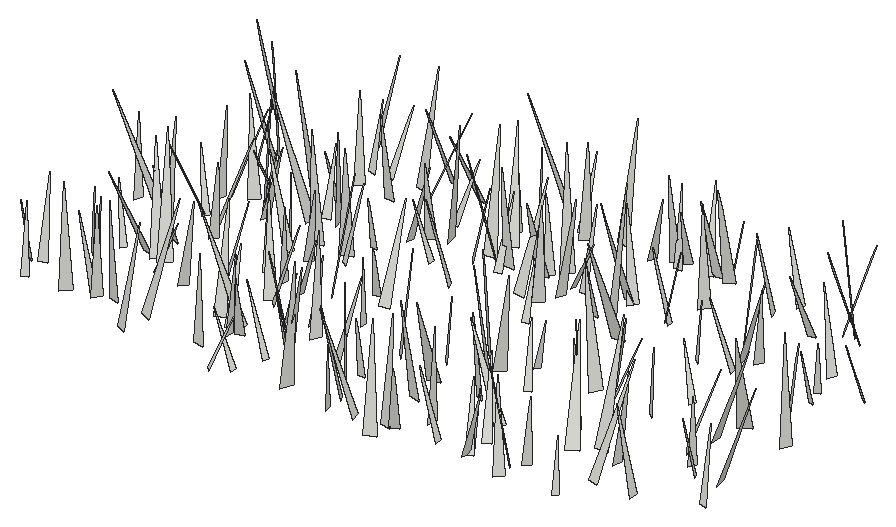
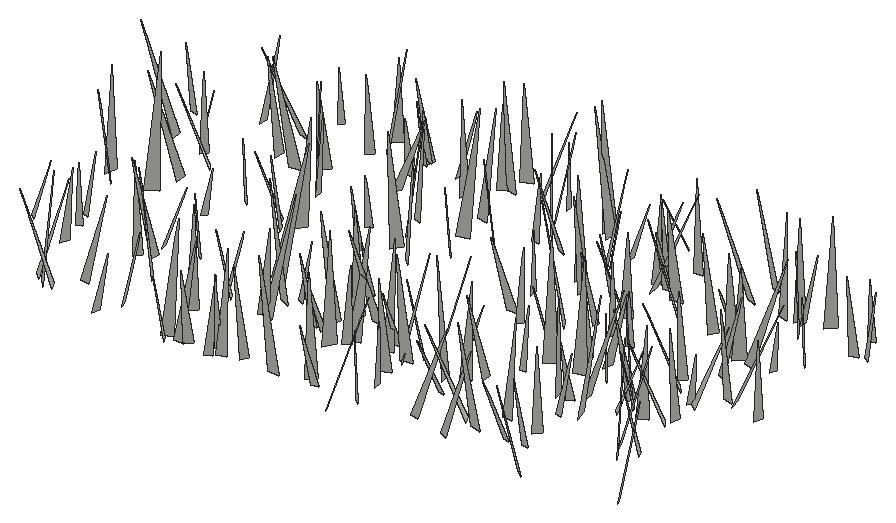
# SketchUp Ruby script. Lengths in inches.
U = 1.inch
M = Sketchup.active_model
def pt(a) = Geom::Point3d.new(a.map { |v| v * U })
def face(e, loops, mat)
  f = e.add_face(loops[0].map { |a| pt(a) })
  loops[1..].each { |l| e.add_face(l.map { |a| pt(a) }).erase! }
  f.material = f.back_material = mat if mat
  f
end
# faces: each face lists its corners as indices into pts; further lists are holes
def faces(e, pts, list, mat = nil) = list.each { |f| face(e, (f[0].is_a?(Array) ? f : [f]).map { |l| l.map { |i| pts[i] } }, mat) }
# xy, xz, yz: faces in a plane at the given z, y or x. An outline is a flat list of corners, or four numbers for a rectangle; further outlines are holes
def ring(l) = l.size == 4 ? [[l[0], l[1]], [l[2], l[1]], [l[2], l[3]], [l[0], l[3]]] : l.each_slice(2).to_a
def flat(e, list, mat, &to3) = list.each { |f| face(e, (f[0].is_a?(Array) ? f : [f]).map { |l| ring(l).map { |u, v| to3.(u, v) } }, mat) }
def xy(e, z, list, mat = nil) = flat(e, list, mat) { |x, y| [x, y, z] }
def xz(e, y, list, mat = nil) = flat(e, list, mat) { |x, z| [x, y, z] }
def yz(e, x, list, mat = nil) = flat(e, list, mat) { |y, z| [x, y, z] }
def lines(e, pts, list) = list.each { |a, b| e.add_line(pt(pts[a]), pt(pts[b])) }
# prism: a flat outline (further loops are holes) pulled along v
def prism(e, loops, v, mat = nil)
  f = face(e, loops, mat); d = Geom::Vector3d.new(v.map { |x| x * U })
  f.pushpull(f.normal.samedirection?(d) ? d.length : -d.length)
end
def box(e, o, s, mat = nil) = prism(e, [[o, [o[0] + s[0], o[1], o[2]], [o[0] + s[0], o[1] + s[1], o[2]], [o[0], o[1] + s[1], o[2]]]], [0, 0, s[2]], mat)
def at(x, y, z, deg = 0) = Geom::Transformation.translation(pt([x, y, z])) * Geom::Transformation.rotation(ORIGIN, Z_AXIS, deg.degrees)
def axes(o, x, y, z) = Geom::Transformation.new([*x, 0, *y, 0, *z, 0, *pt(o).to_a, 1])
def part(name) = M.definitions.add(name)
# library, detail: a bought-in or finely detailed component or shape, given as its bounding box
def library(name, o, s) = part(name).tap { |d| box(d.entities, o, s) }
def detail(e, o, s) = box(e.add_group.entities, o, s)
def put(e, d, t, mat = nil) = e.add_instance(d, t).tap { |i| i.material = mat if mat }
def group(e, t, mat = nil) = e.add_group.tap { |g| g.transformation = t; g.material = mat if mat }.entities
root = M.entities
c1 = part("fur_instance\#9")
p = [[0.8125,0,1.79],[0.67,-0.02,1.48],[0,-0.11,0],[0,0.11,0]]
faces(c1.entities,p,[[0,1,2,3]])
put(root,c1,axes([509.51,356.84,-21.66],[-2.53684,6.34204,1.9532],[6.60869,2.60398,0.12835],[0.60133,-1.86275,6.82939]))
put(root,c1,axes([486.03,357.42,-21.66],[2.19151,2.85606,0.09461],[2.85445,-2.18225,-0.24214],[0.13471,-0.22234,3.59182]))
put(root,c1,axes([510.63,359.85,-21.66],[2.81621,-4.35059,0.38195],[-4.36621,-2.81499,0.12899],[-0.09891,0.39082,5.18093]))
put(root,c1,axes([502.12,358.6,-21.66],[3.8396,0.83392,1.68617],[0.96833,-4.16197,-0.14664],[-1.61273,-0.51356,3.92638]))
put(root,c1,axes([505.58,359.22,-21.66],[-6.60705,-1.5953,0.55499],[-1.61141,6.62494,-0.14037],[0.50631,0.26714,6.79547]))
put(root,c1,axes([488.34,358.98,-21.66],[-3.79909,0.62191,0.11225],[0.62576,3.79759,0.13861],[0.08831,-0.15497,3.84716]))
put(root,c1,axes([526.51,358.57,-21.66],[-4.60516,3.74944,1.60687],[3.84875,4.79672,-0.16237],[1.35183,-0.88372,5.93628]))
put(root,c1,axes([472.625,358.48,-21.66],[2.70818,5.99392,1.73773],[6.22026,-2.74585,-0.22279],[-0.5051,-1.67756,6.57356]))
put(root,c1,axes([534.09,359.27,-21.66],[2.31719,-2.3997,1.71249],[-2.74416,-2.55172,0.13746],[-1.07739,1.33819,3.33302]))
put(root,c1,axes([520.69,360.01,-21.66],[4.88822,-0.89007,0.63341],[-0.87396,-4.92864,-0.18113],[-0.65546,-0.06625,4.96529]))
put(root,c1,axes([495.4,359.7,-21.66],[7.52534,-2.11015,2.94691],[-2.32099,-8.02168,0.183],[-2.78389,0.98374,7.81345]))
put(root,c1,axes([509.59,359.5625,-21.66],[-1.17344,-6.36654,3.3674],[-7.15717,1.41187,0.17527],[0.80444,3.27459,6.4714]))
put(root,c1,axes([516.35,360.58,-21.66],[-4.66446,-0.17714,0.77084],[-0.14932,4.72517,0.1823],[0.77671,-0.15541,4.66426]))
put(root,c1,axes([494.57,360.53,-21.66],[7.78387,0.2727,2.09642],[0.3333,-8.05673,-0.18953],[-2.08764,-0.26953,7.78634]))
put(root,c1,axes([525.74,361.49,-21.66],[4.20893,3.73459,3.7879],[4.59902,-4.98198,-0.19834],[-2.67289,-2.69131,5.62342]))
put(root,c1,axes([501.75,361.46,-21.66],[-4.7875,-3.33897,1.34753],[-3.4677,4.87923,-0.23006],[0.96934,0.96392,5.83232]))
put(root,c1,axes([481.63,361.12,-21.66],[0.33576,5.45677,2.6197],[6.05197,-0.25349,-0.24764],[0.11336,-2.62894,5.46148]))
put(root,c1,axes([520.93,360.85,-21.66],[1.65832,3.59632,1.35209],[3.82471,-1.68517,-0.20869],[-0.36513,-1.31848,3.95475]))
put(root,c1,axes([462.46,361.47,-21.66],[-4.98307,4.13485,3.06586],[4.6284,5.46651,0.15019],[2.25263,-2.08511,6.47344]))
put(root,c1,axes([521.05,360.26,-21.66],[-1.86481,4.13252,0.34952],[4.14724,1.85655,0.17621],[-0.01744,-0.39104,4.53037]))
put(root,c1,axes([456.92,361.08,-21.66],[-1.17354,4.22506,1.16991],[4.38332,1.15287,0.2334],[0.0799,-1.19029,4.3788]))
put(root,c1,axes([466.07,362.47,-21.66],[4.61817,-3.87726,2.02523],[-4.05143,-4.90172,-0.14567],[-1.64942,1.18414,6.02822]))
put(root,c1,axes([527.37,362.58,-21.66],[-2.45808,3.26284,2.53045],[3.74921,2.99751,-0.22312],[1.72995,-1.86016,4.07903]))
put(root,c1,axes([468.05,363.0625,-21.66],[-1.72933,-6.01967,2.37326],[-6.41752,1.90965,0.16749],[0.82719,2.23073,6.26091]))
put(root,c1,axes([465.38,362.79,-21.66],[-4.97388,0.03891,0.99351],[0.0174,5.07103,-0.11152],[0.99411,0.10595,4.97278]))
put(root,c1,axes([513.2,363.39,-21.66],[5.69837,-0.41307,2.53776],[-0.52377,-6.22748,0.16244],[-2.51724,0.36068,5.71101]))
put(root,c1,axes([489.6875,363.09,-21.66],[-4.67921,0.76999,0.1435],[0.76372,4.67821,-0.1991],[0.17382,0.17327,4.73796]))
put(root,c1,axes([454.9,364.58,-21.66],[-2.14945,-3.42966,1.0737],[-3.50191,2.27993,0.27214],[0.80747,0.75821,4.03839]))
put(root,c1,axes([541.13,364.33,-21.66],[-5.71627,0.02456,1.51927],[0.09668,5.9079,0.26822],[1.51639,-0.28405,5.71003]))
put(root,c1,axes([483.88,365.71,-21.66],[1.95757,-4.55386,0.31612],[-4.56359,-1.94437,0.25034],[0.10577,0.38911,4.95045]))
put(root,c1,axes([473.11,362.37,-21.66],[2.96798,6.81466,1.03357],[6.887,-2.97737,-0.1458],[-0.27767,-1.00619,7.4315]))
put(root,c1,axes([499.75,364.73,-21.66],[4.37424,4.04681,2.79179],[4.54542,-4.75288,-0.23239],[-1.87347,-2.08284,5.95454]))
put(root,c1,axes([482.98,364.96,-21.66],[5.23095,-0.44242,1.6949],[-0.413,-5.49862,-0.16069],[-1.70231,-0.02548,5.24716]))
put(root,c1,axes([464.22,365.03,-21.66],[4.38059,2.58911,2.20412],[2.75267,-4.81057,0.18002],[-1.99611,-0.9519,5.08534]))
put(root,c1,axes([508.18,366.46,-21.66],[-1.31696,-6.51866,1.83434],[-6.75362,1.40125,0.13086],[0.49623,1.77078,6.64907]))
put(root,c1,axes([520.74,363.67,-21.66],[-2.1836,4.82414,0.14178],[4.82373,2.17653,0.23433],[-0.15514,-0.2257,5.29014]))
put(root,c1,axes([490.73,366.17,-21.66],[3.77255,3.78798,3.73229],[4.48771,-4.72284,0.25719],[-2.85294,-2.4201,5.33992]))
put(root,c1,axes([456.43,364.95,-21.66],[-1.35199,5.16754,1.66066],[5.39955,1.4549,-0.13134],[0.55327,-1.57128,5.33986]))
put(root,c1,axes([490.39,365.94,-21.66],[-3.18222,-1.83698,0.96818],[-1.93012,3.2701,-0.13938],[0.76583,0.60852,3.67173]))
put(root,c1,axes([500.37,366.75,-21.66],[0.0054,-4.02258,1.09842],[-4.16704,0.03516,0.14925],[0.15324,1.09787,4.01982]))
put(root,c1,axes([483.22,367.07,-21.66],[-7.85705,-0.88135,0.16267],[-0.88597,7.85465,-0.23661],[0.1352,0.25331,7.90278]))
put(root,c1,axes([535.55,364.12,-21.66],[2.14003,7.20036,0.0672],[7.19519,-2.14104,0.27303],[-0.28086,0.01341,7.50668]))
put(root,c1,axes([482.07,366.15,-21.66],[-0.89857,4.82904,0.37817],[4.8418,0.88433,0.21213],[-0.14006,-0.41036,4.90735]))
put(root,c1,axes([496.72,366.71,-21.66],[2.68485,5.08236,0.90598],[5.15716,-2.6868,-0.21076],[-0.23424,-0.9002,5.74408]))
put(root,c1,axes([519.68,367.41,-21.66],[-6.207,1.9177,0.03314],[1.91765,6.20287,0.22937],[-0.03607,-0.22893,6.49244]))
put(root,c1,axes([507.38,370.92,-21.66],[2.10072,-7.09935,0.00934],[-7.09522,-2.09917,0.25546],[0.24231,0.08144,7.39923]))
put(root,c1,axes([548.48,367.56,-21.66],[0.70725,4.81258,1.31899],[4.97344,-0.78845,0.21001],[-0.40688,-1.27212,4.85974]))
put(root,c1,axes([479.67,367.54,-21.66],[-1.61925,6.67608,1.38838],[6.8184,1.60284,0.24489],[0.08425,-1.4073,6.86528]))
put(root,c1,axes([535.05,369.13,-21.66],[5.91491,-0.67607,1.90084],[-0.77835,-6.19702,0.21795],[-1.8613,0.44302,5.94943]))
put(root,c1,axes([459.38,370.02,-21.66],[3.09242,2.58599,1.68004],[2.84079,-3.31463,-0.12697],[-1.19992,-1.18273,4.02918]))
put(root,c1,axes([471.875,370.59,-21.66],[4.94298,-3.20176,1.42299],[-3.34359,-5.04595,0.26096],[-1.0472,0.99819,5.88356]))
put(root,c1,axes([529.19,368.38,-21.66],[-4.20767,6.2047,0.57896],[6.20765,4.23458,-0.26697],[0.54635,-0.32858,7.49209]))
put(root,c1,axes([491,370.375,-21.66],[-5.47966,3.19166,2.7493],[3.39794,6.01513,-0.2105],[2.48986,-1.18473,6.33791]))
put(root,c1,axes([513.71,371.15,-21.66],[-1.84582,-5.09705,1.94608],[-5.40108,1.99766,0.10933],[0.77171,1.78987,5.41987]))
put(root,c1,axes([486.34,370.81,-21.66],[3.55375,0.65284,0.74182],[0.70307,-3.6162,-0.18565],[-0.69441,-0.32026,3.60844]))
put(root,c1,axes([477.64,369.89,-21.66],[4.5925,4.65986,1.11021],[4.70947,-4.6734,0.13435],[-0.87619,-0.69491,6.5412]))
put(root,c1,axes([464.23,373.92,-21.66],[-1.51656,-6.50321,0.08888],[-6.50028,1.51258,-0.24097],[-0.21452,0.14123,6.67335]))
put(root,c1,axes([467.46,371.33,-21.66],[3.69637,0.13401,0.11411],[0.12786,-3.69317,0.19555],[-0.12096,0.19138,3.69362]))
put(root,c1,axes([489.01,372.57,-21.66],[4.9839,-2.53795,0.76874],[-2.53211,-5.04073,-0.2255],[-0.78777,0.14572,5.58834]))
put(root,c1,axes([543.72,372.26,-21.66],[-3.07283,-1.79032,0.75021],[-1.87261,3.10397,-0.26279],[0.51124,0.60869,3.54662]))
put(root,c1,axes([531.77,370.43,-21.66],[-0.24232,8.0833,1.63068],[8.24361,0.27788,-0.15248],[0.20433,-1.625,8.08549]))
put(root,c1,axes([527.19,372.4,-21.66],[-5.46878,-3.64969,2.6695],[-4.02035,5.84198,-0.2491],[2.0696,1.70441,6.57007]))
put(root,c1,axes([546.8,372.83,-21.66],[7.02887,1.41814,0.69885],[1.44367,-7.05544,-0.2028],[-0.64447,-0.3379,7.16763]))
put(root,c1,axes([541.86,373.99,-21.66],[3.93082,-2.70083,1.38603],[-2.7651,-4.12134,-0.18897],[-1.2529,0.6221,4.76552]))
put(root,c1,axes([526.03,373.43,-21.66],[-5.05567,-0.39861,1.84756],[-0.46846,5.37567,-0.1221],[1.83109,0.27472,5.06989]))
put(root,c1,axes([500.86,373.11,-21.66],[4.54729,4.68314,2.12923],[4.88324,-4.82336,0.17985],[-1.61844,-1.39522,6.52513]))
put(root,c1,axes([461.32,373.11,-21.66],[-3.55756,1.9012,0.49829],[1.88183,3.59228,-0.2708],[0.56709,0.00632,4.02461]))
put(root,c1,axes([512.83,374.14,-21.66],[-6.35073,-3.49942,2.22612],[-3.7296,6.59945,-0.26567],[1.81428,1.31702,7.24617]))
put(root,c1,axes([482.47,373.45,-21.66],[3.7464,3.46532,0.67043],[3.46985,-3.79505,0.22613],[-0.64655,-0.28736,5.09832]))
put(root,c1,axes([481.64,373.92,-21.66],[-3.36286,5.21282,1.50099],[5.38655,3.41774,0.19865],[0.64152,-1.37145,6.20023]))
put(root,c1,axes([465.86,373.52,-21.66],[-5.00326,5.02156,1.24961],[5.08502,5.09325,-0.10752],[0.95924,-0.80806,7.08781]))
put(root,c1,axes([466.94,373.46,-21.66],[-4.81371,6.17541,1.55135],[6.27572,4.93015,-0.15223],[1.07597,-1.1279,7.82843]))
put(root,c1,axes([505.83,375.13,-21.66],[3.13173,2.6382,1.54856],[2.8558,-3.31576,-0.12654],[-1.0966,-1.10068,4.0929]))
put(root,c1,axes([493.28,376.03,-21.66],[-3.94466,-0.14605,1.57067],[-0.23954,4.23653,-0.20765],[1.55915,0.28136,3.94189]))
put(root,c1,axes([464.99,377.78,-21.66],[-2.33347,-4.94017,0.88075],[-4.99474,2.38012,0.11709],[0.48332,0.74554,5.4623]))
put(root,c1,axes([511.69,377.36,-21.66],[5.17414,-4.36417,1.70527],[-4.54977,-5.28673,0.27499],[-1.1196,1.31532,6.76329]))
put(root,c1,axes([517,375.77,-21.66],[-1.66344,3.87519,0.54462],[3.91265,1.65754,0.1564],[0.06977,-0.56232,4.21422]))
put(root,c1,axes([483.39,377.17,-21.66],[4.21997,-0.6182,0.41958],[-0.60999,-4.24047,-0.11271],[-0.43142,-0.05127,4.26352]))
put(root,c1,axes([539.4,376.08,-21.66],[4.3993,3.63087,0.47155],[3.65139,-4.40515,-0.14642],[-0.27004,-0.41338,5.70225]))
put(root,c1,axes([480.38,377.96,-21.66],[4.66089,-0.94094,1.87831],[-0.93791,-5.02216,-0.1885],[-1.87983,0.17273,4.75118]))
put(root,c1,axes([508.77,379.15,-21.66],[-4.32305,-4.69404,2.5219],[-5.10648,4.57733,-0.23372],[1.52244,2.02405,6.37716]))
put(root,c1,axes([477.3,378.7,-21.66],[-1.55614,3.71904,0.91385],[3.82438,1.56093,0.15988],[0.20123,-0.90564,4.0283]))
put(root,c1,axes([486.06,379.45,-21.66],[6.38411,4.40631,2.11358],[4.61615,-6.57865,-0.22824],[-1.60436,-1.39477,7.75373]))
put(root,c1,axes([514.53,380.46,-21.66],[2.97768,-2.23657,0.59018],[-2.29034,-2.98547,0.24174],[-0.32391,0.5494,3.71623]))
put(root,c1,axes([531.14,379.95,-21.66],[2.46567,3.17158,1.58955],[3.37143,-2.69731,0.15219],[-1.10413,-1.15357,4.01439]))
put(root,c1,axes([540.26,380.12,-21.66],[6.68807,0.43229,0.66728],[0.41432,-6.71942,0.20043],[-0.67859,0.15798,6.69903]))
put(root,c1,axes([467.89,381.05,-21.66],[3.7544,-3.60472,1.46029],[-3.77286,-3.86843,0.15082],[-0.94444,1.12393,5.20257]))
put(root,c1,axes([490.26,382.14,-21.66],[1.67975,-3.93598,0.16611],[-3.93538,-1.66827,0.26597],[0.17974,0.25696,4.27115]))
put(root,c1,axes([522.85,380.53,-21.66],[-6.40886,3.74132,2.19702],[3.96061,6.64492,0.23769],[1.77143,-1.32114,7.41717]))
put(root,c1,axes([525.56,380.47,-21.66],[3.83341,2.26597,0.28943],[2.28132,-3.82668,-0.25597],[-0.11822,-0.36786,4.44568]))
put(root,c1,axes([459.98,381.63,-21.66],[-7.66892,-1.90839,0.15613],[-1.91216,7.66661,-0.21311],[0.09999,0.24454,7.89993]))
put(root,c1,axes([541.15,384.23,-21.66],[4.3126,-6.65441,0.44802],[-6.65528,-4.32849,-0.22777],[-0.435,0.25174,7.9264]))
put(root,c1,axes([460.99,381.65,-21.66],[1.59622,5.71911,2.00108],[6.0184,-1.73595,0.16062],[-0.70101,-1.88115,5.93551]))
put(root,c1,axes([524.24,382.32,-21.66],[4.12014,1.91723,1.34742],[2.03951,-4.27599,-0.15214],[-1.154,-0.71202,4.54182]))
put(root,c1,axes([479.39,383.64,-21.66],[3.84963,-3.94903,0.87916],[-4.01863,-3.87266,0.20133],[-0.4673,0.77142,5.51126]))
put(root,c1,axes([492.52,380.69,-21.66],[-0.48607,6.36101,0.33267],[6.36907,0.48063,0.1158],[-0.09028,-0.34048,6.37851]))
put(root,c1,axes([455.69,382.9,-21.66],[-4.75498,1.70819,1.94206],[1.76287,5.11453,-0.18234],[1.89256,-0.47231,5.04921]))
put(root,c1,axes([463.16,385.12,-21.66],[-3.18461,-4.17271,0.10236],[-4.17132,3.18622,0.10881],[0.1486,0.01532,5.24799]))
put(root,c1,axes([547.39,383.74,-21.66],[6.19428,-1.57461,3.33029],[-1.87234,-6.95675,0.19327],[-3.17247,1.03131,6.38836]))
put(root,c1,axes([466.87,382.76,-21.66],[4.58247,4.01128,0.43645],[4.00699,-4.60163,0.22113],[-0.47421,-0.12046,6.08609]))
put(root,c1,axes([476.4375,383.78,-21.66],[-5.80582,1.67481,0.45332],[1.66732,5.82342,-0.1609],[0.48013,0.02943,6.04042]))
put(root,c1,axes([463.92,384.56,-21.66],[-3.60805,2.068,0.36238],[2.05277,3.62596,-0.25393],[0.44056,0.04128,4.15092]))
put(root,c1,axes([533.08,384.93,-21.66],[-2.90723,2.3787,0.42473],[2.40963,2.90345,0.23285],[0.1797,-0.4498,3.74913]))
put(root,c1,axes([546.18,385.34,-21.66],[3.88828,4.27161,1.82836],[4.44707,-4.1121,0.14976],[-1.3465,-1.2459,5.77433]))
put(root,c1,axes([481.9375,387.12,-21.66],[3.60415,-6.43604,2.10161],[-6.7075,-3.71823,0.11619],[-0.92131,1.89247,7.37557]))
put(root,c1,axes([474.4375,386.49,-21.66],[2.87799,2.64757,1.74089],[2.94858,-3.09885,-0.16173],[-1.16026,-1.30792,3.90721]))
put(root,c1,axes([477.77,387.0625,-21.66],[1.68119,-6.78383,2.85706],[-7.30642,-1.89388,-0.19753],[-0.89411,2.72073,6.98625]))
put(root,c1,axes([482.83,385.64,-21.66],[2.64907,4.14771,0.84835],[4.17625,-2.72433,0.27885],[-0.69438,-0.56151,4.91358]))
put(root,c1,axes([469.53,388.16,-21.66],[5.0608,-1.8582,0.79428],[-1.91101,-5.09708,0.2516],[-0.65714,0.51221,5.38529]))
put(root,c1,axes([517.55,391.21,-21.66],[0.59961,-8.00132,0.48644],[-8.01433,-0.60861,-0.13198],[-0.1682,0.47514,8.02267]))
put(root,c1,axes([507.09,387.62,-21.66],[-0.85461,3.70026,0.75554],[3.7566,0.91253,-0.21994],[0.38824,-0.68446,3.79129]))
put(root,c1,axes([495.14,389.13,-21.66],[-4.90258,-2.23132,0.87524],[-2.28191,4.95484,-0.15015],[0.73329,0.50088,5.38438]))
put(root,c1,axes([462.8,388.78,-21.66],[5.47635,-0.94494,2.24683],[-1.1073,-5.8869,0.22307],[-2.17142,0.61884,5.55279]))
put(root,c1,axes([483.2,390.41,-21.66],[0.28978,-3.77503,0.68612],[-3.83038,-0.24462,0.27184],[0.22308,0.70349,3.77636]))
put(root,c1,axes([468.47,389.36,-21.66],[-4.89725,-3.9807,3.26033],[-4.56553,5.43754,-0.21877],[2.37312,2.24631,6.30723]))
put(root,c1,axes([468.35,389.17,-21.66],[2.84043,2.51238,0.82611],[2.52394,-2.93724,0.2547],[-0.79009,-0.35083,3.78354]))
put(root,c1,axes([469.16,391.39,-21.66],[-2.85386,-2.94003,0.13695],[-2.93623,2.85714,0.14971],[0.2028,-0.00613,4.09462]))
put(root,c1,axes([473.71,391.01,-21.66],[-7.9003,-1.05971,0.99848],[-1.05239,7.96314,0.1246],[1.0062,0.00826,7.97008]))
put(root,c1,axes([465.95,390.77,-21.66],[-4.07853,4.6775,2.02917],[4.97181,4.22458,0.25488],[1.13033,-1.70436,6.20068]))
put(root,c1,axes([463.3,390.04,-21.66],[4.56753,3.50086,0.36537],[3.49009,-4.58212,0.27435],[-0.45689,-0.00383,5.74831]))
put(root,c1,axes([490.24,391.97,-21.66],[-3.8674,0.14725,0.40736],[0.1724,3.88071,0.23399],[0.39736,-0.25058,3.86312]))
put(root,c1,axes([505.23,392.23,-21.66],[-4.12278,4.06528,3.37823],[4.64279,4.83304,-0.14992],[2.52655,-2.24755,5.78803]))
put(root,c1,axes([476.7,392.24,-21.66],[5.38301,1.51294,2.42188],[1.75431,-5.82988,-0.25732],[-2.2532,-0.92457,5.58566]))
put(root,c1,axes([543.37,393.25,-21.66],[-0.97443,-3.66118,0.75209],[-3.71136,1.03977,0.25308],[0.44234,0.6588,3.78017]))
put(root,c1,axes([527.48,392.79,-21.66],[-2.04031,-2.94511,1.87891],[-3.25881,2.38849,0.20512],[1.25863,1.41005,3.57693]))
put(root,c1,axes([512.32,393.71,-21.66],[-1.30736,-3.53096,1.01989],[-3.67333,1.2908,-0.2398],[0.12042,1.04076,3.75757]))
put(root,c1,axes([532.06,393.42,-21.66],[-4.50006,-1.01814,0.39176],[-1.03948,4.50642,-0.22865],[0.331,0.31016,4.60813]))
put(root,c1,axes([474.9,392.37,-21.66],[-1.60634,4.05647,0.77587],[4.09581,1.67158,-0.25963],[0.53033,-0.623,4.35521]))
put(root,c1,axes([471.78,394.42,-21.66],[-7.67624,-2.38765,2.18106],[-2.53698,7.93,-0.24775],[2.0054,0.89261,8.03519]))
put(root,c1,axes([502.64,392.11,-21.66],[0.72086,7.11073,0.81641],[7.15729,-0.71063,-0.13028],[0.04812,-0.82534,7.14599]))
put(root,c1,axes([485.32,394.32,-21.66],[5.08569,0.11573,0.95874],[0.07501,-5.17107,0.22632],[-0.96278,0.20845,5.08197]))
put(root,c1,axes([502,397.05,-21.66],[2.77965,-6.05851,0.20454],[-6.05263,-2.78627,-0.276],[-0.3362,0.0706,6.66001]))
put(root,c1,axes([486.8125,396.11,-21.66],[3.24454,-4.71501,1.03025],[-4.7617,-3.32972,-0.24278],[-0.78672,0.70811,5.71834]))
put(root,c1,axes([506.35,394.9,-21.66],[6.38697,-1.69717,1.73981],[-1.81592,-6.58358,0.24416],[-1.61547,0.69051,6.6041]))
put(root,c1,axes([473.87,395.83,-21.66],[-0.63245,-3.70623,0.66325],[-3.76509,0.62047,-0.12308],[-0.01169,0.67448,3.75779]))
put(root,c1,axes([542.48,395.51,-21.66],[1.6475,-3.20979,0.84583],[-3.31321,-1.64761,0.20101],[-0.20196,0.8456,3.6023]))
put(root,c1,axes([493.76,394.95,-21.66],[4.05853,2.67005,1.15678],[2.78357,-4.14094,-0.20805],[-0.84796,-0.81387,4.85361]))
put(root,c1,axes([497.67,396.32,-21.66],[0.14601,-6.62439,2.10053],[-6.94709,-0.08453,0.21629],[0.18059,2.1039,6.62247]))
put(root,c1,axes([531.47,395.82,-21.66],[5.98361,0.11352,0.76596],[0.13466,-6.02993,-0.15823],[-0.76252,-0.17402,5.9826]))
put(root,c1,axes([513.71,394.95,-21.66],[3.41828,7.22194,2.57308],[7.56489,-3.63472,0.1519],[-1.24484,-2.25703,7.98861]))
put(root,c1,axes([533.1875,396.69,-21.66],[4.53528,-3.04969,1.17101],[-3.07507,-4.66168,-0.23091],[-1.10265,0.45689,5.46041]))
put(root,c1,axes([495.05,397.33,-21.66],[-4.80805,-4.95386,1.3489],[-5.02147,4.92244,0.17909],[1.0701,0.84054,6.90116]))
put(root,c1,axes([497.5,394.71,-21.66],[-0.4926,4.67354,0.05511],[4.67276,0.49124,0.10792],[-0.10156,-0.0661,4.69819]))
put(root,c1,axes([513.0625,398.69,-21.66],[-2.01035,-7.12989,1.00319],[-7.18316,2.0575,0.22838],[0.49393,0.90254,7.40437]))
put(root,c1,axes([547.67,397.29,-21.66],[-2.17535,-3.01047,0.60266],[-3.06621,2.16789,-0.23847],[0.15643,0.62897,3.70651]))
put(root,c1,axes([463.9,397.43,-21.66],[-6.35383,-3.10693,1.06991],[-3.1587,6.41685,-0.12448],[0.9057,0.58302,7.07168]))
put(root,c1,axes([488.82,397.28,-21.66],[7.15031,1.42356,2.57616],[1.59453,-7.56218,-0.24693],[-2.47399,-0.75958,7.28646]))
put(root,c1,axes([506.3,397.24,-21.66],[3.59656,-0.31618,0.04156],[-0.31764,-3.59357,0.14939],[-0.02828,0.15246,3.60734]))
put(root,c1,axes([519.87,397.48,-21.66],[-4.57594,-0.69447,0.70937],[-0.73517,4.61906,-0.2203],[0.6671,0.32667,4.62309]))
put(root,c1,axes([461.07,397.26,-21.66],[3.50621,1.98379,0.78234],[2.0421,-3.55715,-0.13217],[-0.61424,-0.50223,4.02634]))
put(root,c1,axes([502.26,398,-21.66],[2.60909,-3.89298,2.22887],[-4.24925,-2.97119,-0.21539],[-1.4377,1.71676,4.68148]))
put(root,c1,axes([507.89,396.99,-21.66],[0.83118,5.18677,1.07004],[5.28228,-0.88982,0.21009],[-0.38088,-1.02179,5.24874]))
put(root,c1,axes([519,397.78,-21.66],[-3.23487,-1.73884,2.61208],[-2.22596,3.91581,-0.14997],[2.2117,1.39779,3.66954]))
put(root,c1,axes([494.65,396.99,-21.66],[-1.18605,7.62635,1.82441],[7.84154,1.15487,0.27022],[0.00582,-1.84431,7.7133]))
put(root,c1,axes([513.9,398.4,-21.66],[-4.47005,3.93119,1.60818],[4.11701,4.5843,0.23722],[1.04438,-1.24571,5.94805]))
put(root,c1,axes([462.84,399.07,-21.66],[-5.77727,-4.35757,2.82703],[-4.73437,6.15702,-0.18467],[2.13687,1.8601,7.23403]))
put(root,c1,axes([477.77,400.1,-21.66],[-0.39451,-5.89979,1.57703],[-6.09619,0.47415,0.24879],[0.36204,1.55494,5.90773]))
put(root,c1,axes([528.8,399.64,-21.66],[5.52113,3.74347,2.2115],[4.00437,-5.77059,-0.2291],[-1.6939,-1.44011,6.66663]))
put(root,c1,axes([541.49,399.4,-21.66],[-4.9618,2.41645,1.1014],[2.44275,5.06865,-0.11597],[1.04177,-0.37582,5.51772]))
put(root,c1,axes([503.73,399.41,-21.66],[5.91163,-3.56463,4.13587],[-4.286,-6.80601,0.26026],[-3.38262,2.39395,6.89828]))
put(root,c1,axes([473.07,400.5625,-21.66],[3.99343,-3.31881,2.86458],[-3.84361,-4.5142,0.12826],[-2.10878,1.94301,5.19091]))
put(root,c1,axes([487.09,400.125,-21.66],[1.39427,3.92432,0.17719],[3.92808,-1.39069,-0.10895],[0.04345,-0.20342,4.16322]))
put(root,c1,axes([495.04,400.22,-21.66],[-2.95766,6.66869,1.17233],[6.76114,2.97762,0.11972],[0.36439,-1.12067,7.29416]))
put(root,c1,axes([520.61,402.69,-21.66],[4.6761,-4.10232,2.76945],[-4.45315,-5.14998,-0.1096],[-2.16064,1.73593,6.21956]))
put(root,c1,axes([533.99,405.18,-21.66],[0.26999,-5.16111,0.17986],[-5.16087,-0.27616,-0.17741],[-0.18667,0.17024,5.16512]))
put(root,c1,axes([493.77,403.26,-21.66],[-4.03311,-0.04964,1.55556],[-0.10181,4.31995,-0.1261],[1.55302,0.15428,4.03144]))
put(root,c1,axes([486.14,406.15,-21.66],[-1.09873,-5.30096,0.04279],[-5.29764,1.09638,-0.20521],[-0.19227,0.08352,5.40974]))
put(root,c1,axes([481.14,403.07,-21.66],[5.4364,3.24485,0.19999],[3.25087,-5.4295,-0.27539],[-0.03035,-0.33899,6.32516]))
put(root,c1,axes([472.36,403.68,-21.66],[0.52075,4.40411,1.27547],[4.58416,-0.47433,-0.2338],[0.09203,-1.29345,4.42863]))
put(root,c1,axes([474.73,404.02,-21.66],[0.96438,4.41888,0.40988],[4.43511,-0.94495,-0.24768],[0.15571,-0.45288,4.5161]))
put(root,c1,axes([479.1,404.11,-21.66],[1.99412,7.08431,1.8343],[7.27705,-2.12036,0.27805],[-0.77249,-1.68678,7.35436]))
put(root,c1,axes([538.9,407.34,-21.66],[-4.24041,-4.62675,0.86788],[-4.65391,4.29598,0.16351],[0.70788,0.52807,6.27385]))
put(root,c1,axes([480.99,407.375,-21.66],[-2.16973,-4.86696,0.63571],[-4.9077,2.16207,-0.19771],[0.07681,0.6613,5.32503]))
put(root,c1,axes([456.41,406.79,-21.66],[-5.55068,-3.03255,1.58004],[-3.06213,5.7489,0.27653],[1.52193,0.50669,6.31901]))
put(root,c1,axes([500.48,406.57,-21.66],[3.75494,-4.9741,2.2471],[-5.32599,-3.93562,0.18806],[-1.1937,1.91308,6.22943]))
put(root,c1,axes([527.41,406.52,-21.66],[-4.67685,-1.64881,1.07356],[-1.71505,4.77313,-0.14071],[0.96421,0.49258,4.95698]))
put(root,c1,axes([509.15,407.72,-21.66],[4.77577,-2.2799,0.31782],[-2.26651,-4.78515,-0.26858],[-0.40236,-0.10607,5.28524]))
put(root,c1,axes([519.17,408.95,-21.66],[2.40943,-6.40182,1.38295],[-6.51779,-2.4885,-0.16399],[-0.64358,1.23501,6.83826]))
put(root,c1,axes([493.33,407.46,-21.66],[2.79577,3.11606,1.7882],[3.42019,-3.00212,-0.11591],[-1.09992,-1.41467,4.18482]))
put(root,c1,axes([517.26,409.23,-21.66],[0.8568,-5.86099,0.80486],[-5.91149,-0.87995,-0.11477],[-0.231,0.77949,5.92218]))
put(root,c1,axes([511.58,408.75,-21.66],[1.49133,-6.04191,1.54576],[-6.23212,-1.50337,0.13646],[-0.23383,1.53405,6.22175]))
put(root,c1,axes([512.8125,409.5,-21.66],[2.32528,-3.90872,0.2043],[-3.90658,-2.33236,-0.15975],[-0.24182,0.09371,4.54527]))
put(root,c1,axes([537.51,408.3,-21.66],[-5.07554,-4.81191,2.50581],[-5.17107,5.32884,-0.24106],[1.64121,1.90882,6.98981]))
put(root,c1,axes([512.68,407.89,-21.66],[-0.37436,4.96388,1.61425],[5.21969,0.34743,0.14211],[-0.02763,-1.62026,4.97594]))
put(root,c1,axes([536.22,408.03,-21.66],[5.52496,2.9641,0.73245],[3.00682,-5.54515,-0.24054],[-0.53047,-0.55942,6.26523]))
put(root,c1,axes([499.2,407.65,-21.66],[-0.62067,4.74172,0.56344],[4.77083,0.63973,-0.12835],[0.20124,-0.5417,4.78044]))
put(root,c1,axes([504.53,408.36,-21.66],[0.76042,7.54721,2.45249],[7.93568,-0.724,-0.23253],[-0.00259,-2.46349,7.58186]))
put(root,c1,axes([495.14,410.42,-21.66],[-6.81995,-3.62088,0.84533],[-3.65528,6.85252,-0.13797],[0.68141,0.51893,7.72033]))
put(root,c1,axes([468.87,408.98,-21.66],[3.65147,4.43575,1.22236],[4.5601,-3.69672,-0.20725],[-0.61278,-1.07778,5.74161]))
put(root,c1,axes([516.36,408.79,-21.66],[-2.91757,4.706,0.99504],[4.75363,2.9987,-0.24403],[0.73452,-0.71423,5.53165]))
put(root,c1,axes([518.86,409.94,-21.66],[3.30079,2.00098,0.99665],[2.11543,-3.37049,-0.23912],[-0.72261,-0.72685,3.85253]))
put(root,c1,axes([528.85,409.62,-21.66],[-4.50468,1.1443,0.55643],[1.12699,4.53841,-0.20945],[0.5907,0.0676,4.64302]))
